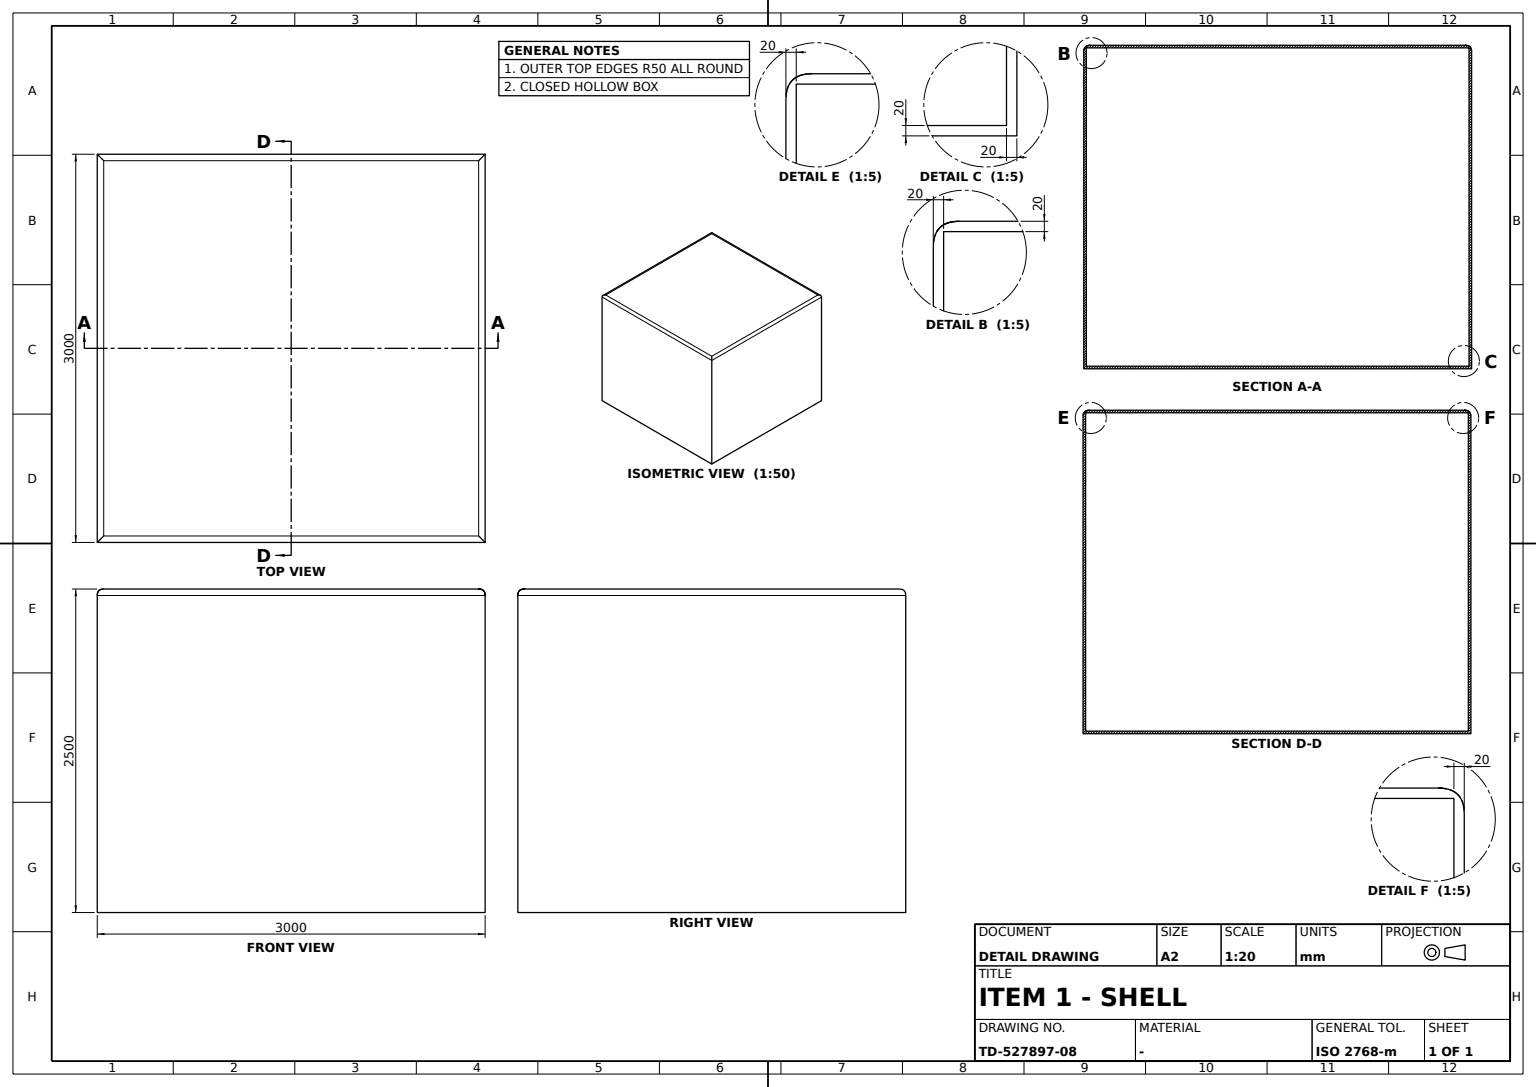
ISO-10303-21;
HEADER;
FILE_DESCRIPTION((''),'2;1');
FILE_NAME('','',(''),(''),'','','');
FILE_SCHEMA(('AUTOMOTIVE_DESIGN'));
ENDSEC;
DATA;
#1=APPLICATION_CONTEXT('');
#2=PRODUCT_CONTEXT('',#1,'mechanical');
#3=PRODUCT('','','',(#2));
#4=PRODUCT_DEFINITION_FORMATION('','',#3);
#5=PRODUCT_DEFINITION_CONTEXT('',#1,'design');
#6=PRODUCT_DEFINITION('','',#4,#5);
#7=PRODUCT_DEFINITION_SHAPE('','',#6);
#8=(LENGTH_UNIT()NAMED_UNIT(*)SI_UNIT(.MILLI.,.METRE.));
#9=(NAMED_UNIT(*)PLANE_ANGLE_UNIT()SI_UNIT($,.RADIAN.));
#10=(NAMED_UNIT(*)SI_UNIT($,.STERADIAN.)SOLID_ANGLE_UNIT());
#11=UNCERTAINTY_MEASURE_WITH_UNIT(LENGTH_MEASURE(0.005),#8,'distance_accuracy_value','');
#12=(GEOMETRIC_REPRESENTATION_CONTEXT(3)GLOBAL_UNCERTAINTY_ASSIGNED_CONTEXT((#11))GLOBAL_UNIT_ASSIGNED_CONTEXT((#8,#9,#10))REPRESENTATION_CONTEXT('',''));
#13=CARTESIAN_POINT('',(1500.,1500.,2450.));
#14=VERTEX_POINT('',#13);
#15=CARTESIAN_POINT('',(1500.,-1500.,2450.));
#16=VERTEX_POINT('',#15);
#17=DIRECTION('',(0.,-1.,0.));
#18=VECTOR('',#17,1000.);
#19=LINE('',#13,#18);
#20=EDGE_CURVE('',#14,#16,#19,.T.);
#21=ORIENTED_EDGE('',*,*,#20,.T.);
#22=CARTESIAN_POINT('',(1500.,-1500.,0.));
#23=VERTEX_POINT('',#22);
#24=DIRECTION('',(0.,0.,1.));
#25=VECTOR('',#24,1000.);
#26=LINE('',#22,#25);
#27=EDGE_CURVE('',#23,#16,#26,.T.);
#28=ORIENTED_EDGE('',*,*,#27,.F.);
#29=CARTESIAN_POINT('',(1500.,1500.,0.));
#30=VERTEX_POINT('',#29);
#31=CARTESIAN_POINT('',(1500.,0.,0.));
#32=LINE('',#31,#18);
#33=EDGE_CURVE('',#30,#23,#32,.T.);
#34=ORIENTED_EDGE('',*,*,#33,.F.);
#35=LINE('',#29,#25);
#36=EDGE_CURVE('',#30,#14,#35,.T.);
#37=ORIENTED_EDGE('',*,*,#36,.T.);
#38=EDGE_LOOP('',(#21,#28,#34,#37));
#39=FACE_BOUND('',#38,.T.);
#40=DIRECTION('',(-1.,0.,0.));
#41=AXIS2_PLACEMENT_3D('',#29,#40,#17);
#42=PLANE('',#41);
#43=ADVANCED_FACE('',(#39),#42,.F.);
#44=CARTESIAN_POINT('',(1450.,-1450.,2500.));
#45=VERTEX_POINT('',#44);
#46=CARTESIAN_POINT('',(-1450.,-1450.,2500.));
#47=VERTEX_POINT('',#46);
#48=CARTESIAN_POINT('',(0.,-1450.,2500.));
#49=DIRECTION('',(1.,0.,0.));
#50=VECTOR('',#49,1000.);
#51=LINE('',#48,#50);
#52=EDGE_CURVE('',#45,#47,#51,.F.);
#53=ORIENTED_EDGE('',*,*,#52,.F.);
#54=CARTESIAN_POINT('',(1450.,1450.,2500.));
#55=VERTEX_POINT('',#54);
#56=CARTESIAN_POINT('',(1450.,0.,2500.));
#57=DIRECTION('',(0.,1.,0.));
#58=VECTOR('',#57,1000.);
#59=LINE('',#56,#58);
#60=EDGE_CURVE('',#55,#45,#59,.F.);
#61=ORIENTED_EDGE('',*,*,#60,.F.);
#62=CARTESIAN_POINT('',(-1450.,1450.,2500.));
#63=VERTEX_POINT('',#62);
#64=CARTESIAN_POINT('',(0.,1450.,2500.));
#65=LINE('',#64,#50);
#66=EDGE_CURVE('',#63,#55,#65,.T.);
#67=ORIENTED_EDGE('',*,*,#66,.F.);
#68=CARTESIAN_POINT('',(-1450.,0.,2500.));
#69=LINE('',#68,#58);
#70=EDGE_CURVE('',#47,#63,#69,.T.);
#71=ORIENTED_EDGE('',*,*,#70,.F.);
#72=EDGE_LOOP('',(#53,#61,#67,#71));
#73=FACE_BOUND('',#72,.T.);
#74=CARTESIAN_POINT('',(0.,0.,2500.));
#75=AXIS2_PLACEMENT_3D('',#74,#24,#49);
#76=PLANE('',#75);
#77=ADVANCED_FACE('',(#73),#76,.T.);
#78=CARTESIAN_POINT('',(-1500.,1500.,0.));
#79=VERTEX_POINT('',#78);
#80=CARTESIAN_POINT('',(-1500.,1500.,2450.));
#81=VERTEX_POINT('',#80);
#82=LINE('',#78,#25);
#83=EDGE_CURVE('',#79,#81,#82,.T.);
#84=ORIENTED_EDGE('',*,*,#83,.F.);
#85=CARTESIAN_POINT('',(-1500.,-1500.,0.));
#86=VERTEX_POINT('',#85);
#87=CARTESIAN_POINT('',(-1500.,0.,0.));
#88=LINE('',#87,#58);
#89=EDGE_CURVE('',#86,#79,#88,.T.);
#90=ORIENTED_EDGE('',*,*,#89,.F.);
#91=CARTESIAN_POINT('',(-1500.,-1500.,2450.));
#92=VERTEX_POINT('',#91);
#93=LINE('',#85,#25);
#94=EDGE_CURVE('',#86,#92,#93,.T.);
#95=ORIENTED_EDGE('',*,*,#94,.T.);
#96=LINE('',#91,#58);
#97=EDGE_CURVE('',#92,#81,#96,.T.);
#98=ORIENTED_EDGE('',*,*,#97,.T.);
#99=EDGE_LOOP('',(#84,#90,#95,#98));
#100=FACE_BOUND('',#99,.T.);
#101=AXIS2_PLACEMENT_3D('',#85,#49,#57);
#102=PLANE('',#101);
#103=ADVANCED_FACE('',(#100),#102,.F.);
#104=CARTESIAN_POINT('',(0.,-1500.,0.));
#105=VECTOR('',#40,1000.);
#106=LINE('',#104,#105);
#107=EDGE_CURVE('',#23,#86,#106,.T.);
#108=ORIENTED_EDGE('',*,*,#107,.F.);
#109=ORIENTED_EDGE('',*,*,#27,.T.);
#110=LINE('',#15,#105);
#111=EDGE_CURVE('',#16,#92,#110,.T.);
#112=ORIENTED_EDGE('',*,*,#111,.T.);
#113=ORIENTED_EDGE('',*,*,#94,.F.);
#114=EDGE_LOOP('',(#108,#109,#112,#113));
#115=FACE_BOUND('',#114,.T.);
#116=AXIS2_PLACEMENT_3D('',#22,#57,#40);
#117=PLANE('',#116);
#118=ADVANCED_FACE('',(#115),#117,.F.);
#119=ORIENTED_EDGE('',*,*,#33,.T.);
#120=ORIENTED_EDGE('',*,*,#107,.T.);
#121=ORIENTED_EDGE('',*,*,#89,.T.);
#122=CARTESIAN_POINT('',(0.,1500.,0.));
#123=LINE('',#122,#50);
#124=EDGE_CURVE('',#79,#30,#123,.T.);
#125=ORIENTED_EDGE('',*,*,#124,.T.);
#126=EDGE_LOOP('',(#119,#120,#121,#125));
#127=FACE_BOUND('',#126,.T.);
#128=CARTESIAN_POINT('',(0.,0.,0.));
#129=AXIS2_PLACEMENT_3D('',#128,#24,#49);
#130=PLANE('',#129);
#131=ADVANCED_FACE('',(#127),#130,.F.);
#132=ORIENTED_EDGE('',*,*,#36,.F.);
#133=ORIENTED_EDGE('',*,*,#124,.F.);
#134=ORIENTED_EDGE('',*,*,#83,.T.);
#135=LINE('',#80,#50);
#136=EDGE_CURVE('',#81,#14,#135,.T.);
#137=ORIENTED_EDGE('',*,*,#136,.T.);
#138=EDGE_LOOP('',(#132,#133,#134,#137));
#139=FACE_BOUND('',#138,.T.);
#140=AXIS2_PLACEMENT_3D('',#78,#17,#49);
#141=PLANE('',#140);
#142=ADVANCED_FACE('',(#139),#141,.F.);
#143=CARTESIAN_POINT('',(1455.035209,-1455.035213,2500.));
#144=CARTESIAN_POINT('',(1462.512371,-1462.512363,2499.451537));
#145=CARTESIAN_POINT('',(1472.266801,-1472.266803,2496.951209));
#146=CARTESIAN_POINT('',(1479.419784,-1479.419781,2493.879868));
#147=CARTESIAN_POINT('',(1486.286184,-1486.286186,2489.146255));
#148=CARTESIAN_POINT('',(1491.636294,-1491.636286,2483.095457));
#149=CARTESIAN_POINT('',(1495.4056,-1495.405603,2476.11697));
#150=CARTESIAN_POINT('',(1497.818467,-1497.818462,2469.439994));
#151=CARTESIAN_POINT('',(1499.558454,-1499.558456,2460.869697));
#152=CARTESIAN_POINT('',(1500.,-1500.,2453.776409));
#153=B_SPLINE_CURVE_WITH_KNOTS('',3,(#44,#143,#144,#145,#146,#147,#148,#149,#150,#151,#152,#15),.UNSPECIFIED.,.F.,.F.,(4,1,1,1,1,1,1,1,1,4),(0.,32.043895829,48.065843744,64.087791659,80.109739573,96.131687488,104.142661445,112.153635403,120.16460936,128.175583317),.UNSPECIFIED.);
#154=EDGE_CURVE('',#16,#45,#153,.F.);
#155=ORIENTED_EDGE('',*,*,#154,.T.);
#156=ORIENTED_EDGE('',*,*,#52,.T.);
#157=CARTESIAN_POINT('',(-1455.035213,-1455.035209,2500.));
#158=CARTESIAN_POINT('',(-1462.512363,-1462.512371,2499.451537));
#159=CARTESIAN_POINT('',(-1472.266803,-1472.266801,2496.951209));
#160=CARTESIAN_POINT('',(-1479.419781,-1479.419784,2493.879868));
#161=CARTESIAN_POINT('',(-1486.286186,-1486.286184,2489.146255));
#162=CARTESIAN_POINT('',(-1491.636286,-1491.636294,2483.095457));
#163=CARTESIAN_POINT('',(-1495.405603,-1495.4056,2476.11697));
#164=CARTESIAN_POINT('',(-1497.818462,-1497.818467,2469.439995));
#165=CARTESIAN_POINT('',(-1499.558456,-1499.558454,2460.869697));
#166=CARTESIAN_POINT('',(-1500.,-1500.,2453.776409));
#167=B_SPLINE_CURVE_WITH_KNOTS('',3,(#46,#157,#158,#159,#160,#161,#162,#163,#164,#165,#166,#91),.UNSPECIFIED.,.F.,.F.,(4,1,1,1,1,1,1,1,1,4),(0.,32.043895822,48.065843732,64.087791643,80.109739554,96.131687465,104.14266142,112.153635375,120.164609331,128.175583286),.UNSPECIFIED.);
#168=EDGE_CURVE('',#92,#47,#167,.F.);
#169=ORIENTED_EDGE('',*,*,#168,.F.);
#170=ORIENTED_EDGE('',*,*,#111,.F.);
#171=EDGE_LOOP('',(#155,#156,#169,#170));
#172=FACE_BOUND('',#171,.T.);
#173=CARTESIAN_POINT('',(1518.,-1500.,2450.));
#174=CARTESIAN_POINT('',(1518.,-1500.,2470.));
#175=CARTESIAN_POINT('',(1518.,-1495.,2485.));
#176=CARTESIAN_POINT('',(1518.,-1485.,2495.));
#177=CARTESIAN_POINT('',(1518.,-1470.,2500.));
#178=CARTESIAN_POINT('',(1518.,-1450.,2500.));
#179=CARTESIAN_POINT('',(910.8,-1500.,2450.));
#180=CARTESIAN_POINT('',(910.8,-1500.,2470.));
#181=CARTESIAN_POINT('',(910.8,-1495.,2485.));
#182=CARTESIAN_POINT('',(910.8,-1485.,2495.));
#183=CARTESIAN_POINT('',(910.8,-1470.,2500.));
#184=CARTESIAN_POINT('',(910.8,-1450.,2500.));
#185=CARTESIAN_POINT('',(303.6,-1500.,2450.));
#186=CARTESIAN_POINT('',(303.6,-1500.,2470.));
#187=CARTESIAN_POINT('',(303.6,-1495.,2485.));
#188=CARTESIAN_POINT('',(303.6,-1485.,2495.));
#189=CARTESIAN_POINT('',(303.6,-1470.,2500.));
#190=CARTESIAN_POINT('',(303.6,-1450.,2500.));
#191=CARTESIAN_POINT('',(-303.6,-1500.,2450.));
#192=CARTESIAN_POINT('',(-303.6,-1500.,2470.));
#193=CARTESIAN_POINT('',(-303.6,-1495.,2485.));
#194=CARTESIAN_POINT('',(-303.6,-1485.,2495.));
#195=CARTESIAN_POINT('',(-303.6,-1470.,2500.));
#196=CARTESIAN_POINT('',(-303.6,-1450.,2500.));
#197=CARTESIAN_POINT('',(-910.8,-1500.,2450.));
#198=CARTESIAN_POINT('',(-910.8,-1500.,2470.));
#199=CARTESIAN_POINT('',(-910.8,-1495.,2485.));
#200=CARTESIAN_POINT('',(-910.8,-1485.,2495.));
#201=CARTESIAN_POINT('',(-910.8,-1470.,2500.));
#202=CARTESIAN_POINT('',(-910.8,-1450.,2500.));
#203=CARTESIAN_POINT('',(-1518.,-1500.,2450.));
#204=CARTESIAN_POINT('',(-1518.,-1500.,2470.));
#205=CARTESIAN_POINT('',(-1518.,-1495.,2485.));
#206=CARTESIAN_POINT('',(-1518.,-1485.,2495.));
#207=CARTESIAN_POINT('',(-1518.,-1470.,2500.));
#208=CARTESIAN_POINT('',(-1518.,-1450.,2500.));
#209=B_SPLINE_SURFACE_WITH_KNOTS('',5,5,((#173,#174,#175,#176,#177,#178),(#179,#180,#181,#182,#183,#184),(#185,#186,#187,#188,#189,#190),(#191,#192,#193,#194,#195,#196),(#197,#198,#199,#200,#201,#202),(#203,#204,#205,#206,#207,#208)),.SURF_OF_LINEAR_EXTRUSION.,.F.,.F.,.F.,(6,6),(6,6),(0.281216667,3.308783333),(0.,0.098),.PIECEWISE_BEZIER_KNOTS.);
#210=ADVANCED_FACE('',(#172),#209,.F.);
#211=ORIENTED_EDGE('',*,*,#154,.F.);
#212=ORIENTED_EDGE('',*,*,#20,.F.);
#213=CARTESIAN_POINT('',(1500.,1500.,2453.776409));
#214=CARTESIAN_POINT('',(1499.558454,1499.558456,2460.869697));
#215=CARTESIAN_POINT('',(1497.818467,1497.818462,2469.439995));
#216=CARTESIAN_POINT('',(1495.4056,1495.405603,2476.11697));
#217=CARTESIAN_POINT('',(1491.636294,1491.636286,2483.095457));
#218=CARTESIAN_POINT('',(1486.286184,1486.286186,2489.146255));
#219=CARTESIAN_POINT('',(1479.419784,1479.419781,2493.879868));
#220=CARTESIAN_POINT('',(1472.266801,1472.266803,2496.951209));
#221=CARTESIAN_POINT('',(1462.512371,1462.512363,2499.451537));
#222=CARTESIAN_POINT('',(1455.035209,1455.035213,2500.));
#223=B_SPLINE_CURVE_WITH_KNOTS('',3,(#13,#213,#214,#215,#216,#217,#218,#219,#220,#221,#222,#54),.UNSPECIFIED.,.F.,.F.,(4,1,1,1,1,1,1,1,1,4),(0.,8.010973956,16.021947911,24.032921867,32.043895823,48.065843734,64.087791646,80.109739557,96.131687469,128.175583291),.UNSPECIFIED.);
#224=EDGE_CURVE('',#14,#55,#223,.T.);
#225=ORIENTED_EDGE('',*,*,#224,.T.);
#226=ORIENTED_EDGE('',*,*,#60,.T.);
#227=EDGE_LOOP('',(#211,#212,#225,#226));
#228=FACE_BOUND('',#227,.T.);
#229=CARTESIAN_POINT('',(1500.,1518.,2450.));
#230=CARTESIAN_POINT('',(1500.,1518.,2470.));
#231=CARTESIAN_POINT('',(1495.,1518.,2485.));
#232=CARTESIAN_POINT('',(1485.,1518.,2495.));
#233=CARTESIAN_POINT('',(1470.,1518.,2500.));
#234=CARTESIAN_POINT('',(1450.,1518.,2500.));
#235=CARTESIAN_POINT('',(1500.,910.8,2450.));
#236=CARTESIAN_POINT('',(1500.,910.8,2470.));
#237=CARTESIAN_POINT('',(1495.,910.8,2485.));
#238=CARTESIAN_POINT('',(1485.,910.8,2495.));
#239=CARTESIAN_POINT('',(1470.,910.8,2500.));
#240=CARTESIAN_POINT('',(1450.,910.8,2500.));
#241=CARTESIAN_POINT('',(1500.,303.6,2450.));
#242=CARTESIAN_POINT('',(1500.,303.6,2470.));
#243=CARTESIAN_POINT('',(1495.,303.6,2485.));
#244=CARTESIAN_POINT('',(1485.,303.6,2495.));
#245=CARTESIAN_POINT('',(1470.,303.6,2500.));
#246=CARTESIAN_POINT('',(1450.,303.6,2500.));
#247=CARTESIAN_POINT('',(1500.,-303.6,2450.));
#248=CARTESIAN_POINT('',(1500.,-303.6,2470.));
#249=CARTESIAN_POINT('',(1495.,-303.6,2485.));
#250=CARTESIAN_POINT('',(1485.,-303.6,2495.));
#251=CARTESIAN_POINT('',(1470.,-303.6,2500.));
#252=CARTESIAN_POINT('',(1450.,-303.6,2500.));
#253=CARTESIAN_POINT('',(1500.,-910.8,2450.));
#254=CARTESIAN_POINT('',(1500.,-910.8,2470.));
#255=CARTESIAN_POINT('',(1495.,-910.8,2485.));
#256=CARTESIAN_POINT('',(1485.,-910.8,2495.));
#257=CARTESIAN_POINT('',(1470.,-910.8,2500.));
#258=CARTESIAN_POINT('',(1450.,-910.8,2500.));
#259=CARTESIAN_POINT('',(1500.,-1518.,2450.));
#260=CARTESIAN_POINT('',(1500.,-1518.,2470.));
#261=CARTESIAN_POINT('',(1495.,-1518.,2485.));
#262=CARTESIAN_POINT('',(1485.,-1518.,2495.));
#263=CARTESIAN_POINT('',(1470.,-1518.,2500.));
#264=CARTESIAN_POINT('',(1450.,-1518.,2500.));
#265=B_SPLINE_SURFACE_WITH_KNOTS('',5,5,((#229,#230,#231,#232,#233,#234),(#235,#236,#237,#238,#239,#240),(#241,#242,#243,#244,#245,#246),(#247,#248,#249,#250,#251,#252),(#253,#254,#255,#256,#257,#258),(#259,#260,#261,#262,#263,#264)),.SURF_OF_LINEAR_EXTRUSION.,.F.,.F.,.F.,(6,6),(6,6),(0.281216667,3.308783333),(0.,0.098),.PIECEWISE_BEZIER_KNOTS.);
#266=ADVANCED_FACE('',(#228),#265,.F.);
#267=ORIENTED_EDGE('',*,*,#66,.T.);
#268=ORIENTED_EDGE('',*,*,#224,.F.);
#269=ORIENTED_EDGE('',*,*,#136,.F.);
#270=CARTESIAN_POINT('',(-1455.035209,1455.035213,2500.));
#271=CARTESIAN_POINT('',(-1462.512371,1462.512363,2499.451537));
#272=CARTESIAN_POINT('',(-1472.266801,1472.266803,2496.951209));
#273=CARTESIAN_POINT('',(-1479.419784,1479.419781,2493.879868));
#274=CARTESIAN_POINT('',(-1486.286184,1486.286186,2489.146255));
#275=CARTESIAN_POINT('',(-1491.636294,1491.636286,2483.095457));
#276=CARTESIAN_POINT('',(-1495.4056,1495.405603,2476.11697));
#277=CARTESIAN_POINT('',(-1497.818467,1497.818462,2469.439995));
#278=CARTESIAN_POINT('',(-1499.558454,1499.558456,2460.869697));
#279=CARTESIAN_POINT('',(-1500.,1500.,2453.776409));
#280=B_SPLINE_CURVE_WITH_KNOTS('',3,(#62,#270,#271,#272,#273,#274,#275,#276,#277,#278,#279,#80),.UNSPECIFIED.,.F.,.F.,(4,1,1,1,1,1,1,1,1,4),(0.,32.043895823,48.065843735,64.087791646,80.109739558,96.131687469,104.142661425,112.153635381,120.164609337,128.175583292),.UNSPECIFIED.);
#281=EDGE_CURVE('',#81,#63,#280,.F.);
#282=ORIENTED_EDGE('',*,*,#281,.T.);
#283=EDGE_LOOP('',(#267,#268,#269,#282));
#284=FACE_BOUND('',#283,.T.);
#285=CARTESIAN_POINT('',(-1518.,1500.,2450.));
#286=CARTESIAN_POINT('',(-1518.,1500.,2470.));
#287=CARTESIAN_POINT('',(-1518.,1495.,2485.));
#288=CARTESIAN_POINT('',(-1518.,1485.,2495.));
#289=CARTESIAN_POINT('',(-1518.,1470.,2500.));
#290=CARTESIAN_POINT('',(-1518.,1450.,2500.));
#291=CARTESIAN_POINT('',(-910.8,1500.,2450.));
#292=CARTESIAN_POINT('',(-910.8,1500.,2470.));
#293=CARTESIAN_POINT('',(-910.8,1495.,2485.));
#294=CARTESIAN_POINT('',(-910.8,1485.,2495.));
#295=CARTESIAN_POINT('',(-910.8,1470.,2500.));
#296=CARTESIAN_POINT('',(-910.8,1450.,2500.));
#297=CARTESIAN_POINT('',(-303.6,1500.,2450.));
#298=CARTESIAN_POINT('',(-303.6,1500.,2470.));
#299=CARTESIAN_POINT('',(-303.6,1495.,2485.));
#300=CARTESIAN_POINT('',(-303.6,1485.,2495.));
#301=CARTESIAN_POINT('',(-303.6,1470.,2500.));
#302=CARTESIAN_POINT('',(-303.6,1450.,2500.));
#303=CARTESIAN_POINT('',(303.6,1500.,2450.));
#304=CARTESIAN_POINT('',(303.6,1500.,2470.));
#305=CARTESIAN_POINT('',(303.6,1495.,2485.));
#306=CARTESIAN_POINT('',(303.6,1485.,2495.));
#307=CARTESIAN_POINT('',(303.6,1470.,2500.));
#308=CARTESIAN_POINT('',(303.6,1450.,2500.));
#309=CARTESIAN_POINT('',(910.8,1500.,2450.));
#310=CARTESIAN_POINT('',(910.8,1500.,2470.));
#311=CARTESIAN_POINT('',(910.8,1495.,2485.));
#312=CARTESIAN_POINT('',(910.8,1485.,2495.));
#313=CARTESIAN_POINT('',(910.8,1470.,2500.));
#314=CARTESIAN_POINT('',(910.8,1450.,2500.));
#315=CARTESIAN_POINT('',(1518.,1500.,2450.));
#316=CARTESIAN_POINT('',(1518.,1500.,2470.));
#317=CARTESIAN_POINT('',(1518.,1495.,2485.));
#318=CARTESIAN_POINT('',(1518.,1485.,2495.));
#319=CARTESIAN_POINT('',(1518.,1470.,2500.));
#320=CARTESIAN_POINT('',(1518.,1450.,2500.));
#321=B_SPLINE_SURFACE_WITH_KNOTS('',5,5,((#285,#286,#287,#288,#289,#290),(#291,#292,#293,#294,#295,#296),(#297,#298,#299,#300,#301,#302),(#303,#304,#305,#306,#307,#308),(#309,#310,#311,#312,#313,#314),(#315,#316,#317,#318,#319,#320)),.SURF_OF_LINEAR_EXTRUSION.,.F.,.F.,.F.,(6,6),(6,6),(0.281216667,3.308783333),(0.,0.098),.PIECEWISE_BEZIER_KNOTS.);
#322=ADVANCED_FACE('',(#284),#321,.F.);
#323=ORIENTED_EDGE('',*,*,#97,.F.);
#324=ORIENTED_EDGE('',*,*,#168,.T.);
#325=ORIENTED_EDGE('',*,*,#70,.T.);
#326=ORIENTED_EDGE('',*,*,#281,.F.);
#327=EDGE_LOOP('',(#323,#324,#325,#326));
#328=FACE_BOUND('',#327,.T.);
#329=CARTESIAN_POINT('',(-1500.,-1518.,2450.));
#330=CARTESIAN_POINT('',(-1500.,-1518.,2470.));
#331=CARTESIAN_POINT('',(-1495.,-1518.,2485.));
#332=CARTESIAN_POINT('',(-1485.,-1518.,2495.));
#333=CARTESIAN_POINT('',(-1470.,-1518.,2500.));
#334=CARTESIAN_POINT('',(-1450.,-1518.,2500.));
#335=CARTESIAN_POINT('',(-1500.,-910.8,2450.));
#336=CARTESIAN_POINT('',(-1500.,-910.8,2470.));
#337=CARTESIAN_POINT('',(-1495.,-910.8,2485.));
#338=CARTESIAN_POINT('',(-1485.,-910.8,2495.));
#339=CARTESIAN_POINT('',(-1470.,-910.8,2500.));
#340=CARTESIAN_POINT('',(-1450.,-910.8,2500.));
#341=CARTESIAN_POINT('',(-1500.,-303.6,2450.));
#342=CARTESIAN_POINT('',(-1500.,-303.6,2470.));
#343=CARTESIAN_POINT('',(-1495.,-303.6,2485.));
#344=CARTESIAN_POINT('',(-1485.,-303.6,2495.));
#345=CARTESIAN_POINT('',(-1470.,-303.6,2500.));
#346=CARTESIAN_POINT('',(-1450.,-303.6,2500.));
#347=CARTESIAN_POINT('',(-1500.,303.6,2450.));
#348=CARTESIAN_POINT('',(-1500.,303.6,2470.));
#349=CARTESIAN_POINT('',(-1495.,303.6,2485.));
#350=CARTESIAN_POINT('',(-1485.,303.6,2495.));
#351=CARTESIAN_POINT('',(-1470.,303.6,2500.));
#352=CARTESIAN_POINT('',(-1450.,303.6,2500.));
#353=CARTESIAN_POINT('',(-1500.,910.8,2450.));
#354=CARTESIAN_POINT('',(-1500.,910.8,2470.));
#355=CARTESIAN_POINT('',(-1495.,910.8,2485.));
#356=CARTESIAN_POINT('',(-1485.,910.8,2495.));
#357=CARTESIAN_POINT('',(-1470.,910.8,2500.));
#358=CARTESIAN_POINT('',(-1450.,910.8,2500.));
#359=CARTESIAN_POINT('',(-1500.,1518.,2450.));
#360=CARTESIAN_POINT('',(-1500.,1518.,2470.));
#361=CARTESIAN_POINT('',(-1495.,1518.,2485.));
#362=CARTESIAN_POINT('',(-1485.,1518.,2495.));
#363=CARTESIAN_POINT('',(-1470.,1518.,2500.));
#364=CARTESIAN_POINT('',(-1450.,1518.,2500.));
#365=B_SPLINE_SURFACE_WITH_KNOTS('',5,5,((#329,#330,#331,#332,#333,#334),(#335,#336,#337,#338,#339,#340),(#341,#342,#343,#344,#345,#346),(#347,#348,#349,#350,#351,#352),(#353,#354,#355,#356,#357,#358),(#359,#360,#361,#362,#363,#364)),.SURF_OF_LINEAR_EXTRUSION.,.F.,.F.,.F.,(6,6),(6,6),(0.281216667,3.308783333),(0.,0.098),.PIECEWISE_BEZIER_KNOTS.);
#366=ADVANCED_FACE('',(#328),#365,.F.);
#367=CLOSED_SHELL('',(#43,#77,#103,#118,#131,#142,#210,#266,#322,#366));
#368=CARTESIAN_POINT('',(1480.,1480.,20.));
#369=VERTEX_POINT('',#368);
#370=CARTESIAN_POINT('',(1480.,-1480.,20.));
#371=VERTEX_POINT('',#370);
#372=CARTESIAN_POINT('',(1480.,0.,20.));
#373=LINE('',#372,#18);
#374=EDGE_CURVE('',#369,#371,#373,.T.);
#375=ORIENTED_EDGE('',*,*,#374,.T.);
#376=CARTESIAN_POINT('',(1480.,-1480.,2480.));
#377=VERTEX_POINT('',#376);
#378=CARTESIAN_POINT('',(1480.,-1480.,0.));
#379=LINE('',#378,#25);
#380=EDGE_CURVE('',#371,#377,#379,.T.);
#381=ORIENTED_EDGE('',*,*,#380,.T.);
#382=CARTESIAN_POINT('',(1480.,1480.,2480.));
#383=VERTEX_POINT('',#382);
#384=CARTESIAN_POINT('',(1480.,0.,2480.));
#385=LINE('',#384,#18);
#386=EDGE_CURVE('',#383,#377,#385,.T.);
#387=ORIENTED_EDGE('',*,*,#386,.F.);
#388=CARTESIAN_POINT('',(1480.,1480.,0.));
#389=LINE('',#388,#25);
#390=EDGE_CURVE('',#369,#383,#389,.T.);
#391=ORIENTED_EDGE('',*,*,#390,.F.);
#392=EDGE_LOOP('',(#375,#381,#387,#391));
#393=FACE_BOUND('',#392,.T.);
#394=AXIS2_PLACEMENT_3D('',#388,#40,#17);
#395=PLANE('',#394);
#396=ADVANCED_FACE('',(#393),#395,.T.);
#397=CARTESIAN_POINT('',(-1480.,-1480.,2480.));
#398=VERTEX_POINT('',#397);
#399=CARTESIAN_POINT('',(-1480.,1480.,2480.));
#400=VERTEX_POINT('',#399);
#401=CARTESIAN_POINT('',(-1480.,0.,2480.));
#402=LINE('',#401,#58);
#403=EDGE_CURVE('',#398,#400,#402,.T.);
#404=ORIENTED_EDGE('',*,*,#403,.T.);
#405=CARTESIAN_POINT('',(0.,1480.,2480.));
#406=LINE('',#405,#50);
#407=EDGE_CURVE('',#400,#383,#406,.T.);
#408=ORIENTED_EDGE('',*,*,#407,.T.);
#409=ORIENTED_EDGE('',*,*,#386,.T.);
#410=CARTESIAN_POINT('',(0.,-1480.,2480.));
#411=LINE('',#410,#105);
#412=EDGE_CURVE('',#377,#398,#411,.T.);
#413=ORIENTED_EDGE('',*,*,#412,.T.);
#414=EDGE_LOOP('',(#404,#408,#409,#413));
#415=FACE_BOUND('',#414,.T.);
#416=CARTESIAN_POINT('',(0.,0.,2480.));
#417=AXIS2_PLACEMENT_3D('',#416,#24,#49);
#418=PLANE('',#417);
#419=ADVANCED_FACE('',(#415),#418,.F.);
#420=ORIENTED_EDGE('',*,*,#403,.F.);
#421=CARTESIAN_POINT('',(-1480.,-1480.,20.));
#422=VERTEX_POINT('',#421);
#423=CARTESIAN_POINT('',(-1480.,-1480.,0.));
#424=LINE('',#423,#25);
#425=EDGE_CURVE('',#422,#398,#424,.T.);
#426=ORIENTED_EDGE('',*,*,#425,.F.);
#427=CARTESIAN_POINT('',(-1480.,1480.,20.));
#428=VERTEX_POINT('',#427);
#429=CARTESIAN_POINT('',(-1480.,0.,20.));
#430=LINE('',#429,#58);
#431=EDGE_CURVE('',#422,#428,#430,.T.);
#432=ORIENTED_EDGE('',*,*,#431,.T.);
#433=CARTESIAN_POINT('',(-1480.,1480.,0.));
#434=LINE('',#433,#25);
#435=EDGE_CURVE('',#428,#400,#434,.T.);
#436=ORIENTED_EDGE('',*,*,#435,.T.);
#437=EDGE_LOOP('',(#420,#426,#432,#436));
#438=FACE_BOUND('',#437,.T.);
#439=AXIS2_PLACEMENT_3D('',#423,#49,#57);
#440=PLANE('',#439);
#441=ADVANCED_FACE('',(#438),#440,.T.);
#442=ORIENTED_EDGE('',*,*,#380,.F.);
#443=CARTESIAN_POINT('',(0.,-1480.,20.));
#444=LINE('',#443,#105);
#445=EDGE_CURVE('',#371,#422,#444,.T.);
#446=ORIENTED_EDGE('',*,*,#445,.T.);
#447=ORIENTED_EDGE('',*,*,#425,.T.);
#448=ORIENTED_EDGE('',*,*,#412,.F.);
#449=EDGE_LOOP('',(#442,#446,#447,#448));
#450=FACE_BOUND('',#449,.T.);
#451=AXIS2_PLACEMENT_3D('',#378,#57,#40);
#452=PLANE('',#451);
#453=ADVANCED_FACE('',(#450),#452,.T.);
#454=ORIENTED_EDGE('',*,*,#374,.F.);
#455=CARTESIAN_POINT('',(0.,1480.,20.));
#456=LINE('',#455,#50);
#457=EDGE_CURVE('',#428,#369,#456,.T.);
#458=ORIENTED_EDGE('',*,*,#457,.F.);
#459=ORIENTED_EDGE('',*,*,#431,.F.);
#460=ORIENTED_EDGE('',*,*,#445,.F.);
#461=EDGE_LOOP('',(#454,#458,#459,#460));
#462=FACE_BOUND('',#461,.T.);
#463=CARTESIAN_POINT('',(0.,0.,20.));
#464=AXIS2_PLACEMENT_3D('',#463,#24,#49);
#465=PLANE('',#464);
#466=ADVANCED_FACE('',(#462),#465,.T.);
#467=ORIENTED_EDGE('',*,*,#407,.F.);
#468=ORIENTED_EDGE('',*,*,#435,.F.);
#469=ORIENTED_EDGE('',*,*,#457,.T.);
#470=ORIENTED_EDGE('',*,*,#390,.T.);
#471=EDGE_LOOP('',(#467,#468,#469,#470));
#472=FACE_BOUND('',#471,.T.);
#473=AXIS2_PLACEMENT_3D('',#433,#17,#49);
#474=PLANE('',#473);
#475=ADVANCED_FACE('',(#472),#474,.T.);
#476=CLOSED_SHELL('',(#396,#419,#441,#453,#466,#475));
#477=ORIENTED_CLOSED_SHELL('',*,#476,.F.);
#478=BREP_WITH_VOIDS('',#367,(#477));
#479=ADVANCED_BREP_SHAPE_REPRESENTATION('',(#478),#12);
#480=SHAPE_DEFINITION_REPRESENTATION(#7,#479);
ENDSEC;
END-ISO-10303-21;
